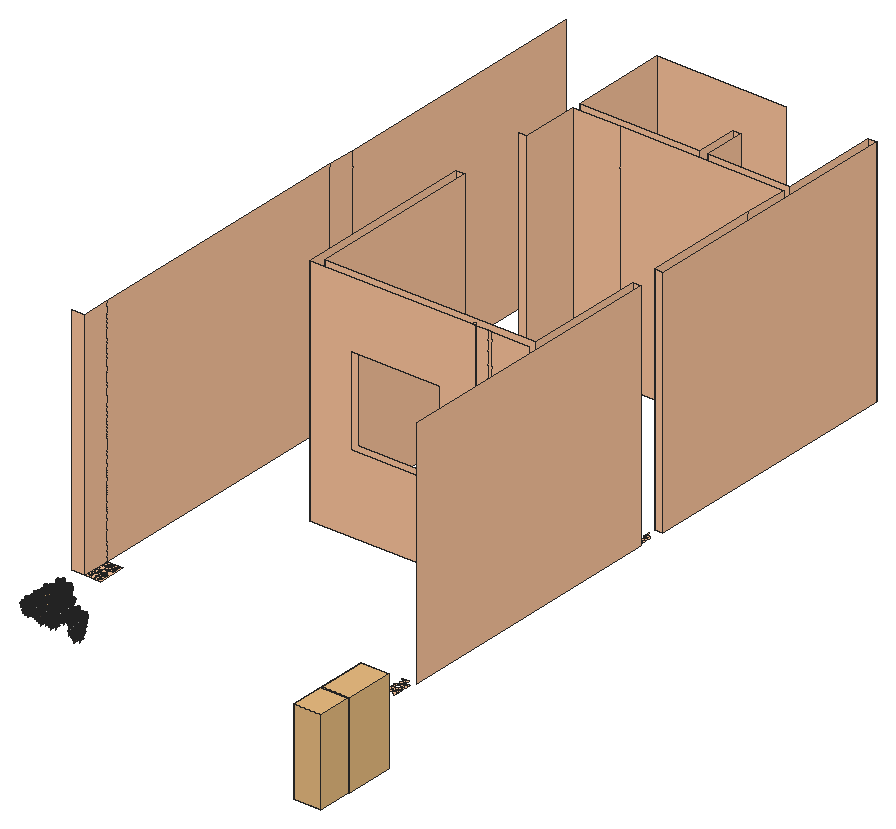
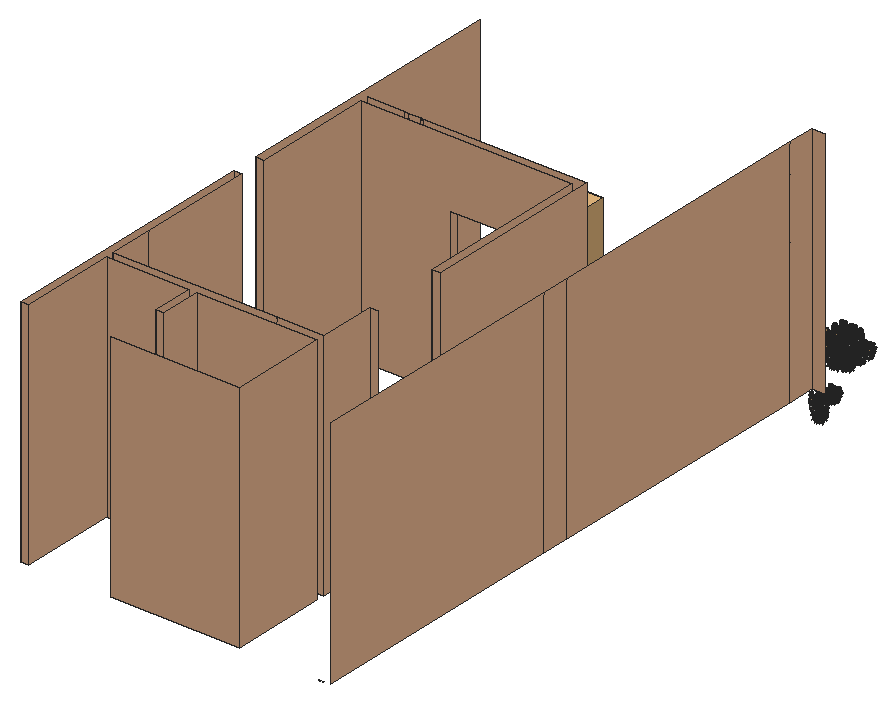
# SketchUp Ruby script. Lengths in inches.
U = 1.inch
M = Sketchup.active_model
def pt(a) = Geom::Point3d.new(a.map { |v| v * U })
def face(e, loops, mat)
  f = e.add_face(loops[0].map { |a| pt(a) })
  loops[1..].each { |l| e.add_face(l.map { |a| pt(a) }).erase! }
  f.material = f.back_material = mat if mat
  f
end
# faces: each face lists its corners as indices into pts; further lists are holes
def faces(e, pts, list, mat = nil) = list.each { |f| face(e, (f[0].is_a?(Array) ? f : [f]).map { |l| l.map { |i| pts[i] } }, mat) }
# xy, xz, yz: faces in a plane at the given z, y or x. An outline is a flat list of corners, or four numbers for a rectangle; further outlines are holes
def ring(l) = l.size == 4 ? [[l[0], l[1]], [l[2], l[1]], [l[2], l[3]], [l[0], l[3]]] : l.each_slice(2).to_a
def flat(e, list, mat, &to3) = list.each { |f| face(e, (f[0].is_a?(Array) ? f : [f]).map { |l| ring(l).map { |u, v| to3.(u, v) } }, mat) }
def xy(e, z, list, mat = nil) = flat(e, list, mat) { |x, y| [x, y, z] }
def xz(e, y, list, mat = nil) = flat(e, list, mat) { |x, z| [x, y, z] }
def yz(e, x, list, mat = nil) = flat(e, list, mat) { |y, z| [x, y, z] }
def lines(e, pts, list) = list.each { |a, b| e.add_line(pt(pts[a]), pt(pts[b])) }
# prism: a flat outline (further loops are holes) pulled along v
def prism(e, loops, v, mat = nil)
  f = face(e, loops, mat); d = Geom::Vector3d.new(v.map { |x| x * U })
  f.pushpull(f.normal.samedirection?(d) ? d.length : -d.length)
end
def box(e, o, s, mat = nil) = prism(e, [[o, [o[0] + s[0], o[1], o[2]], [o[0] + s[0], o[1] + s[1], o[2]], [o[0], o[1] + s[1], o[2]]]], [0, 0, s[2]], mat)
def at(x, y, z, deg = 0) = Geom::Transformation.translation(pt([x, y, z])) * Geom::Transformation.rotation(ORIGIN, Z_AXIS, deg.degrees)
def axes(o, x, y, z) = Geom::Transformation.new([*x, 0, *y, 0, *z, 0, *pt(o).to_a, 1])
def part(name) = M.definitions.add(name)
# library, detail: a bought-in or finely detailed component or shape, given as its bounding box
def library(name, o, s) = part(name).tap { |d| box(d.entities, o, s) }
def detail(e, o, s) = box(e.add_group.entities, o, s)
def put(e, d, t, mat = nil) = e.add_instance(d, t).tap { |i| i.material = mat if mat }
def group(e, t, mat = nil) = e.add_group.tap { |g| g.transformation = t; g.material = mat if mat }.entities
root = M.entities
M.materials.add("Vegetation_Bark_Crabapple").color = [91, 75, 65]
M.materials.add("[Color A02]1").color = [252, 197, 157]
M.materials.add("pollen").color = [217, 178, 104]
c1 = library("House+plant_10",[-33.59,-33.81,-21.29],[25.63,26.45,46.04])
c2 = part("Plane.002")
p = [[-2.92,82.99,124.67],[-2.92,-0.79,0],[2.92,-0.79,0],[2.92,82.99,124.67],[2.92,149.28,292.15],[-2.92,149.28,292.15],
  [2.92,182.43,464.87],[-2.92,182.43,464.87]]
faces(c2.entities,p,[[0,1,2,3],[3,4,5,0],[4,6,7,5]],"Vegetation_Bark_Crabapple")
c3 = part("Plane.003")
p = [[-13.75,10.1875,13.53],[-8.85,45.75,19.16],[-0.05,76.91,20.56],[0.09,-0.03,-0.02],[7.48,49.37,17.16],[14.16,9.16,9.9]]
faces(c3.entities,p,[[0,1,2,3],[4,5,3,2]])
c4 = part("Flower-123")
p = [[0.126,0.257,0.449],[0.155,0.204,0.548],[0.127,0.213,0.555],[0.093,0.267,0.458],[0.188,0.133,0.622],[0.183,0.129,0.631],
  [0.175,0.131,0.633],[0.165,0.14,0.628]]
faces(c4.entities,p,[[0,1,2,3],[1,4,5,6,7,2]],"pollen")
detail(c4.entities,[0,0,0],[0.33,0.41,0.7])
c5 = part("Group\#22")
put(c5.entities,c2,axes([0.24,0.01,0.18],[0.00584,-0.00173,-0.00142],[0.00119,0.00873,-0.00832],[0.00331,0.00566,0.01028]))
put(c5.entities,c3,axes([1.52,3.22,2.1875],[-0.00804,0.00596,-0.00897],[-0.00946,-0.00546,0.00721],[-0.0004,0.00943,0.00985]))
put(c5.entities,c3,axes([1.32,2.77,1.78],[0.01256,0.00031,-0.00351],[-0.00251,0.0076,-0.01232],[0.00145,0.0104,0.00911]))
put(c5.entities,c3,axes([1.78,3.75,2.82],[0.00359,0.00823,-0.01047],[-0.01158,0.00445,-0.0007],[0.0027,0.00817,0.01092]))
put(c5.entities,c3,axes([0.88,1.77,1.02],[0.01086,-0.00723,-0.00215],[0.00311,0.00724,-0.01286],[0.00676,0.00828,0.00937]))
put(c5.entities,c3,axes([1.72,3.66,2.68],[-0.00696,-0.00525,0.00789],[0.00768,-0.00731,0.00284],[0.00323,0.00607,0.01024]))
put(c5.entities,c3,axes([0.98,1.92,1.1],[-0.00641,-0.00676,0.01252],[0.01063,-0.00886,0.00097],[0.00617,0.00824,0.01132]))
put(c5.entities,c3,axes([1.42,3.04,1.99],[0.00101,-0.00541,0.01232],[0.01133,-0.00105,-0.00207],[0.00173,0.0101,0.00638]))
put(c5.entities,c3,axes([0.59,1,0.65],[0.0051,-0.00438,-0.01381],[-0.00968,0.00594,-0.00813],[0.00732,0.01091,-0.00112]))
put(c5.entities,c3,axes([1.1,2.28,1.42],[0.00541,0.00553,-0.01038],[-0.00976,0.00548,-0.00323],[0.00278,0.00847,0.00887]))
put(c5.entities,c3,axes([0.66,1.2,0.69],[0.00787,-0.0076,0.01038],[0.01088,0.00189,-0.01021],[0.00343,0.01143,0.00859]))
put(c5.entities,c3,axes([1,2.02,1.23],[-0.00332,0.0113,-0.00638],[-0.00988,0.0009,0.01004],[0.00758,0.00613,0.01028]))
put(c5.entities,c3,axes([1.58,3.35,2.32],[0.00647,0.00472,-0.01261],[-0.01005,0.00792,-0.00326],[0.0053,0.00927,0.0092]))
put(c5.entities,c3,axes([1.62,3.49,2.49],[0.0094,-0.00757,0.00183],[0.00666,0.00678,-0.00925],[0.00388,0.00669,0.01145]))
put(c5.entities,c3,axes([1.21,2.52,1.61],[-0.01302,0.00172,-0.00109],[-0.0017,-0.00726,0.01324],[0.00092,0.01085,0.00902]))
put(c5.entities,c3,axes([1.125,2.36,1.48],[0.00721,-0.01079,0.00269],[0.00807,0.00338,-0.01201],[0.0075,0.00674,0.01032]))
put(c5.entities,c3,axes([1.9,4,3.09],[0.00001,-0.00487,0.01359],[0.01166,-0.00316,-0.0017],[0.00346,0.01068,0.00569]))
put(c5.entities,c4,axes([2.27,4.3,3.3125],[-0.76505,0.00149,-0.64397],[-0.61285,-0.30881,0.72736],[-0.19778,0.95112,0.23716]))
put(c5.entities,c3,axes([0.67,1.42,0.8125],[0.00418,-0.00177,-0.01289],[-0.00136,0.01117,-0.00294],[0.01063,0.00213,0.0047]))
put(c5.entities,c3,axes([0.36,1.36,0.75],[0.00559,0.00872,-0.00936],[-0.00135,0.00895,0.0112],[0.01154,-0.00318,0.00584]))
put(c5.entities,c3,axes([1.13,1.46,0.92],[0.00037,0.00449,-0.01599],[-0.00588,0.01192,0.00478],[0.01254,0.00546,0.00271]))
put(c5.entities,c4,axes([1.91,4.52,3.45],[-0.75636,-0.57556,0.31088],[0.59252,-0.80417,-0.04724],[0.27718,0.14847,0.94928]))
put(c5.entities,c4,axes([2.12,4.17,3.27],[0.01541,0.99987,-0.00371],[-0.66505,0.01302,0.74668],[0.74664,-0.00904,0.66517]))
put(c5.entities,c4,axes([2.05,4.17,3.1875],[0.05514,0.99835,0.01633],[-0.20485,-0.0047,0.97878],[0.97724,-0.05731,0.20425]))
put(c5.entities,c4,axes([1.95,4.53,3.51],[-0.67965,-0.57263,0.45843],[0.47474,-0.81981,-0.32021],[0.55919,0,0.82904]))
put(c5.entities,c4,axes([2.12,4.37,3.18],[-0.03684,0.90233,0.42946],[-0.20892,-0.42721,0.87968],[0.97724,-0.05731,0.20425]))
put(c5.entities,c4,axes([1.99,3.97,3.47],[0.82904,0,-0.55919],[0,1,0],[0.55919,0,0.82904]))
put(c5.entities,c4,axes([2,3.97,3.43],[0.66131,0,0.75011],[0,1,0],[-0.75011,0,0.66131]))
put(c5.entities,c4,axes([2.28,4.28,3.48],[-0.2877,-0.35709,-0.88866],[-0.91973,-0.15572,0.36033],[-0.26705,0.921,-0.28363]))
put(c5.entities,c4,axes([1.95,4.53,3.46],[-0.85707,-0.51463,-0.02405],[0.51016,-0.85429,0.09964],[-0.07183,0.07313,0.99473]))
put(c5.entities,c4,axes([1.98,4.0625,3.66],[0.10005,0.76886,0.63153],[0.20466,0.60524,-0.76928],[-0.97371,0.20622,-0.0968]))
put(c5.entities,c4,axes([2.21,4.21,3.28],[0.01107,0.99991,-0.00785],[-0.71534,0.01341,0.69865],[0.69869,-0.00211,0.71542]))
put(c5.entities,c4,axes([1.86,4.48,3.42],[-0.09798,-0.20201,0.97447],[0.64597,-0.75778,-0.09214],[0.75705,0.62045,0.20474]))
put(c5.entities,c4,at(2.25,4.35,3.46,120))
put(c5.entities,c4,at(2.02,3.96,3.47))
put(c5.entities,c4,axes([2.1875,4.32,3.26],[-0.2678,0.91122,0.31298],[-0.60895,-0.41181,0.67793],[0.74664,-0.00904,0.66517]))
put(c5.entities,c4,axes([2.03,4.02,3.45],[0.99756,0,-0.06976],[0,1,0],[0.06976,0,0.99756]))
put(c5.entities,c4,axes([2.05,3.99,3.41],[0.19766,0,0.98027],[0,1,0],[-0.98027,0,0.19766]))
put(c5.entities,c4,axes([2.1,4.34,3.72],[-0.09883,0.86603,-0.49014],[-0.17118,-0.5,-0.84894],[-0.98027,0,0.19766]))
put(c5.entities,c4,axes([2.18,4.47,3.53],[0.15137,-0.29348,-0.9439],[-0.69645,-0.7093,0.10885],[-0.70146,0.64091,-0.31176]))
put(c5.entities,c4,axes([2.27,4.23,3.62],[-0.07449,0.99629,-0.04301],[-0.86282,-0.08601,-0.49815],[-0.5,0,0.86603]))
put(c5.entities,c4,axes([1.9,4.51,3.47],[-0.18374,-0.30318,0.93505],[0.54752,-0.82159,-0.1588],[0.81637,0.48278,0.31695]))
put(c5.entities,c4,axes([2.34,4.27,3.47],[-0.11925,0.65296,-0.74794],[-0.99139,-0.11938,0.05384],[-0.05413,0.74792,0.66158]))
put(c5.entities,c4,axes([2.03,4,3.41],[0.86603,0,0.5],[0,1,0],[-0.5,0,0.86603]))
put(c5.entities,c4,axes([1.77,4.36,3.36],[-0.17823,-0.16506,0.97005],[0.98053,-0.11233,0.16104],[0.08239,0.97987,0.18187]))
put(c5.entities,c4,axes([2.2,4.25,3.24],[-0.61909,0.78366,0.05103],[-0.23541,-0.24718,0.93994],[0.74921,0.56989,0.33751]))
put(c5.entities,c4,axes([2.1,4.2,3.19],[-0.58355,0.81023,0.05471],[0.17622,0.06058,0.98249],[0.79273,0.58297,-0.17813]))
put(c5.entities,c4,axes([1.78,4.42,3.35],[-0.12701,-0.00833,0.99187],[0.91049,-0.39772,0.11325],[0.39354,0.91747,0.05809]))
put(c5.entities,c4,axes([1.97,4.33,3.18],[-0.45394,0.75959,0.46579],[0.40685,-0.28839,0.86678],[0.79273,0.58297,-0.17813]))
put(c5.entities,c4,axes([2.2,4.22,3.68],[0.6255,-0.22092,-0.74829],[-0.6737,0.33082,-0.66082],[0.39354,0.91747,0.05809]))
put(c5.entities,c4,axes([2.2,4.05,3.41],[0.46326,0.30792,0.83101],[-0.67387,0.7314,0.10465],[-0.57558,-0.60847,0.54632]))
put(c5.entities,c4,axes([2.09,4.46,3.69],[-0.81522,0.47946,-0.32488],[-0.06426,-0.63237,-0.772],[-0.57558,-0.60847,0.54632]))
put(c5.entities,c4,axes([1.79,4.38,3.33],[-0.28578,-0.47426,0.83271],[0.95001,-0.02622,0.31111],[-0.12572,0.88,0.45804]))
put(c5.entities,c4,axes([2.17,4.34,3.73],[-0.71122,0.70221,0.03278],[-0.40358,-0.36968,-0.83693],[-0.57558,-0.60847,0.54632]))
put(c5.entities,c4,axes([2.2,4.2,3.3],[-0.66528,0.3275,-0.67093],[-0.55383,0.38617,0.73766],[0.50067,0.86233,-0.07553]))
put(c5.entities,c4,axes([1.76,4.3,3.4],[0.04081,0.76243,0.64579],[0.98982,-0.11906,0.07802],[0.13637,0.63603,-0.75952]))
put(c5.entities,c4,axes([2.13,4.49,3.52],[-0.95264,0.30339,0.02075],[-0.30229,-0.93732,-0.17336],[-0.03315,-0.17142,0.98464]))
put(c5.entities,c4,axes([2.25,4,3.45],[0.70641,0.60197,-0.37232],[-0.62885,0.77519,0.06021],[0.32487,0.1916,0.92615]))
put(c5.entities,c4,axes([2.11,4.21,3.23],[-0.81906,0.48983,-0.29868],[-0.18829,0.26227,0.94645],[0.54194,0.83143,-0.12259]))
put(c5.entities,c4,axes([2.2,4.23,3.61],[0.73847,0.26741,-0.61899],[-0.6737,0.33082,-0.66082],[0.02806,0.90501,0.42446]))
put(c5.entities,c4,axes([2.22,4.11,3.4],[0.1134,-0.03757,0.99284],[-0.67387,0.7314,0.10465],[-0.7301,-0.68091,0.05762]))
put(c5.entities,c4,axes([2.01,4.35,3.75],[-0.64029,0.6522,-0.40579],[0.23873,-0.33316,-0.91215],[-0.7301,-0.68091,0.05762]))
put(c5.entities,c4,axes([2.21,4.39,3.67],[-0.72493,0.6869,0.0515],[-0.56238,-0.54702,-0.62008],[-0.39776,-0.47848,0.78285]))
put(c5.entities,c4,axes([1.76,4.37,3.375],[0.04655,0.66582,0.74466],[0.96165,-0.23158,0.14695],[0.27029,0.70926,-0.65107]))
put(c5.entities,c4,axes([2.25,4.43,3.28],[-0.5104,-0.48462,-0.71038],[-0.65311,-0.31894,0.68683],[-0.55942,0.81451,-0.15373]))
put(c5.entities,c4,axes([2.28,4.65,3.33],[-0.5104,-0.48462,-0.71038],[-0.65311,-0.31894,0.68683],[-0.55942,0.81451,-0.15373]))
c6 = part("Group\#23")
put(c6.entities,c5,axes([5.13,2.49,1.91],[-0.108,0.99415,0],[-0.70297,-0.07637,0.70711],[0.70297,0.07637,0.70711]))
put(c6.entities,c5,axes([5.13,2.49,1.08],[-0.108,0.99415,0],[-0.70297,-0.07637,0.70711],[0.70297,0.07637,0.70711]))
put(c6.entities,c5,axes([4.47,2.97,0.4375],[-0.60599,-0.79547,0],[0.56248,-0.4285,0.70711],[-0.56248,0.4285,0.70711]))
put(c6.entities,c5,axes([4.94,2.86,-0.05],[0.00524,-0.99999,0],[0.7071,0.0037,0.70711],[-0.7071,-0.0037,0.70711]))
put(c6.entities,c5,axes([2.93,5.37,1.01],[-0.68962,0.72417,0],[-0.51207,-0.48763,0.70711],[0.51207,0.48763,0.70711]))
put(c6.entities,c5,axes([2.93,4.82,-0.05],[-0.98823,0.15299,0],[-0.10818,-0.69878,0.70711],[0.10818,0.69878,0.70711]))
put(c6.entities,c5,axes([6.18,5.29,1.13],[1,0,0],[0,0.70711,0.70711],[0,-0.70711,0.70711]))
put(c6.entities,c5,axes([3.49,6.03,1.01],[-0.108,0.99415,0],[-0.70297,-0.07637,0.70711],[0.70297,0.07637,0.70711]))
put(c6.entities,c5,axes([6.37,4.16,-0.13],[0.94495,-0.32722,0],[0.23138,0.66818,0.70711],[-0.23138,-0.66818,0.70711]))
put(c6.entities,c5,axes([5.84,5.86,0.11],[0.79441,0.60738,0],[-0.42948,0.56174,0.70711],[0.42948,-0.56174,0.70711]))
put(c6.entities,c5,axes([4.7,6.09,0.1875],[0.25882,0.96593,0],[-0.68301,0.18301,0.70711],[0.68301,-0.18301,0.70711]))
put(c6.entities,c5,axes([3.28,3.87,0.07],[-0.96456,-0.26387,0],[0.18659,-0.68205,0.70711],[-0.18659,0.68205,0.70711]))
put(c6.entities,c5,axes([5.96,3.21,1.01],[0.54902,-0.83581,0],[0.59101,0.38822,0.70711],[-0.59101,-0.38822,0.70711]))
put(c6.entities,c5,axes([4.45,5.31,1.53],[-0.0715,-0.99744,0],[0.7053,-0.05056,0.70711],[-0.7053,0.05056,0.70711]))
put(c6.entities,c5,axes([3.99,3.86,0.1875],[0.00524,-0.99999,0],[0.7071,0.0037,0.70711],[-0.7071,-0.0037,0.70711]))
put(c6.entities,c5,axes([3.84,4.21,0.1875],[-0.60599,-0.79547,0],[0.56248,-0.4285,0.70711],[-0.56248,0.4285,0.70711]))
put(c6.entities,c5,axes([4.45,5.67,0.1875],[-0.0715,-0.99744,0],[0.7053,-0.05056,0.70711],[-0.7053,0.05056,0.70711]))
put(c6.entities,c5,axes([4.68,4.3,0.1875],[0.54902,-0.83581,0],[0.59101,0.38822,0.70711],[-0.59101,-0.38822,0.70711]))
put(c6.entities,c5,axes([3.9,4.47,0.1875],[-0.96456,-0.26387,0],[0.18659,-0.68205,0.70711],[-0.18659,0.68205,0.70711]))
put(c6.entities,c5,axes([5.41,4.87,0.1875],[0.25882,0.96593,0],[-0.68301,0.18301,0.70711],[0.68301,-0.18301,0.70711]))
put(c6.entities,c5,axes([4.68,3.97,0.1875],[0.79441,0.60738,0],[-0.42948,0.56174,0.70711],[0.42948,-0.56174,0.70711]))
put(c6.entities,c5,axes([5.06,3.625,0.1875],[0.94495,-0.32722,0],[0.23138,0.66818,0.70711],[-0.23138,-0.66818,0.70711]))
put(c6.entities,c5,axes([4.64,4.71,0.1875],[-0.108,0.99415,0],[-0.70297,-0.07637,0.70711],[0.70297,0.07637,0.70711]))
put(c6.entities,c5,axes([5.34,4.26,0.1875],[1,0,0],[0,0.70711,0.70711],[0,-0.70711,0.70711]))
put(c6.entities,c5,axes([4.02,5.27,0.1875],[-0.98823,0.15299,0],[-0.10818,-0.69878,0.70711],[0.10818,0.69878,0.70711]))
put(c6.entities,c5,axes([4.38,5.37,0.1875],[-0.68962,0.72417,0],[-0.51207,-0.48763,0.70711],[0.51207,0.48763,0.70711]))
c7 = part("Kukka-altaaat")
put(c7.entities,c6,at(36.02,12.82,2.28))
put(c7.entities,c6,at(36.02,19.85,2.28))
put(c7.entities,c6,at(36.02,7.07,2.28))
put(c7.entities,c6,at(41.52,7.07,2.28))
put(c7.entities,c6,at(41.52,12.76,2.28))
put(c7.entities,c6,at(34.29,32.17,-7.59))
xy(root,-0.11,[[[7.86,46.0625,16.85,61.13],[15.83,48.22,15.65,48.4,15.83,48.6,15.83,49.99,15.65,50.17,15.83,50.37,15.83,51.76,15.65,51.95,14.77,51.05,15.65,50.17,13.91,48.37,13.02,49.26,12.13,50.14,11.25,51.02,10.375,51.9,11.25,52.8,12.13,51.92,13.01,52.8125,13.89,53.71,13.01,54.58,12.13,55.46,13.01,56.36,13.89,55.48,13.01,54.58,13.89,53.71,15.65,51.95,15.83,52.14],[11.25,52.8,10.375,53.67,9.5,54.55,10.39,55.43,11.28,56.32,12.13,55.46,11.25,54.57,10.39,55.43,9.5,54.55,8.87,53.91,8.87,60.12,9.25,60.12,9.5,59.86,8.87,59.23,8.87,58.73,9.5,58.09,8.87,57.46,8.87,56.95,9.5,56.32,8.87,55.6875,8.87,55.18,9.5,54.55,10.375,53.67,11.25,54.57,12.13,53.69],[8.87,47.08,8.87,48.09,9.5,47.46,9.12,47.08,9.88,47.08,9.5,47.46,10.375,48.35,11.27,47.46,10.9,47.08],[11.28,56.32,10.39,57.21,11.28,58.09,12.16,57.21],[13.01,56.36,12.16,57.21,13.05,58.09,13.89,57.25],[9.5,51.01,8.87,51.63,8.87,52.14,9.5,52.78,10.375,51.9],[14.77,58.15,13.93,58.98,14.82,59.86,15.65,59.04],[12.67,47.08,13.04,47.46,13.43,47.08],[14.82,59.86,14.57,60.12,15.07,60.12]],[8.87,47.08,9.12,47.08,9.5,47.46,8.87,48.09],[9.88,47.08,10.9,47.08,11.27,47.46,10.375,48.35,9.5,49.23,10.375,50.13,11.25,49.25,12.13,50.14,11.25,51.02,10.375,50.13,9.5,51.01,8.87,51.63,8.87,50.37,9.5,51.01,8.87,50.37,8.87,49.86,9.5,49.23,10.375,50.13,11.25,49.25,12.15,48.36,13.04,47.46,13.91,48.37,14.8,47.47,14.44,47.08,13.43,47.08,13.04,47.46,12.67,47.08,15.83,47.08,15.83,48.22,14.78,49.27,13.91,48.37,13.02,49.26,12.15,48.36,11.25,49.25,10.375,48.35,9.5,47.46],[9.88,47.08,10.9,47.08,11.27,47.46,10.375,48.35,9.5,47.46],[12.67,47.08,13.43,47.08,13.04,47.46],
  [14.44,47.08,15.2,47.08,14.8,47.47],[15.2,47.08,15.83,47.08,15.83,48.22,15.65,48.4,14.8,47.47],[174.25,47.08,174.88,47.08,174.88,48.22,174.7,48.4,173.82,49.27,172.95,48.37,172.07,49.26,171.18,50.14,170.3,49.25,171.19,48.36,172.07,49.26,172.94,50.15,173.82,49.27,174.7,48.4,173.85,47.47],[13.04,47.46,13.91,48.37,13.02,49.26,12.15,48.36],[14.8,47.47,15.65,48.4,13.9,50.15,14.77,51.05,13.89,51.93,13.01,52.8125,12.13,51.92,13.9,50.15,13.02,49.26,13.91,48.37],
  [15.83,48.22,15.83,48.6,15.65,48.4],[15.83,48.22,15.83,48.6,15.65,48.4],[10.375,48.35,11.25,49.25,10.375,50.13,9.5,49.23],[169.42,48.35,170.3,49.25,169.42,50.13,168.54,49.23],[171.19,48.36,172.07,49.26,171.18,50.14,170.3,49.25],
  [172.95,48.37,173.82,49.27,172.94,50.15,172.07,49.26],[8.87,48.6,8.87,49.86,9.5,49.23,10.375,50.13,9.5,51.01,8.87,50.37,8.87,49.86,9.5,49.23],[8.87,48.6,9.5,49.23,8.87,49.86],[11.25,49.25,12.13,50.14,11.25,51.02,10.375,50.13],[13.02,49.26,13.9,50.15,13.01,51.04,13.89,51.93,14.77,52.83,15.65,53.72,15.83,53.91,15.83,60.12,15.07,60.12,14.82,59.86,15.65,59.04,15.83,59.23,15.83,58.85,15.65,59.04,14.77,58.15,13.89,57.25,13.05,58.09,13.93,58.98,14.82,59.86,14.57,60.12,11.53,60.12,11.28,59.86,10.39,58.98,9.5,58.09,10.39,57.21,9.5,56.32,8.87,56.95,8.87,55.6875,9.5,56.32,10.39,57.21,11.28,58.09,10.39,58.98,9.5,59.86,9.76,60.12,9.25,60.12,9.5,59.86,10.39,58.98,11.28,58.09,12.16,58.98,11.28,59.86,13.05,58.09,12.16,57.21,13.01,56.36,13.89,57.25,15.65,55.49,14.77,54.6,13.89,55.48,14.77,56.37,15.65,55.49,15.83,55.6875,15.83,55.31,15.65,55.49,14.77,54.6,15.65,53.72,14.77,52.83,15.65,51.95,14.77,51.05,13.89,51.93,13.01,51.04,12.13,50.14],
  [13.02,49.26,13.9,50.15,13.01,51.04,12.13,50.14],[14.78,49.27,15.65,50.17,14.77,51.05,13.9,50.15],[173.82,49.27,174.69,50.17,173.82,51.05,172.94,50.15],[15.83,49.99,15.83,50.37,15.65,50.17],[174.88,49.99,174.69,50.17,174.88,50.37,174.88,51.76,174.69,51.95,173.82,51.05,172.93,51.93,172.06,51.04,172.94,50.15,173.82,51.05,174.69,51.95,174.88,52.14],
  [169.42,50.13,170.3,51.02,169.42,51.9,168.54,51.01,167.91,50.37,167.91,51.63,168.54,51.01],[12.13,50.14,13.01,51.04,12.13,51.92,11.25,51.02],[171.18,50.14,172.06,51.04,171.18,51.92,170.3,51.02],[8.87,50.37,9.5,51.01,8.87,51.63],[9.5,51.01,10.375,51.9,9.5,52.78,8.87,52.14,8.87,51.63],
  [11.25,51.02,12.13,51.92,11.25,52.8,10.375,51.9],[170.3,51.02,171.18,51.92,170.3,52.8,169.42,51.9],[172.06,51.04,172.93,51.93,172.06,52.8125,171.18,51.92],[14.77,51.05,15.65,51.95,14.77,52.83,13.89,51.93],[15.83,51.76,15.83,52.14,15.65,51.95],
  [169.42,51.9,170.3,52.8,169.42,53.67,168.54,52.78],[13.89,51.93,14.77,52.83,13.89,53.71,13.01,52.8125],[172.93,51.93,173.8125,52.83,172.93,53.71,172.06,52.8125],[8.87,52.14,9.5,52.78,10.375,53.67,11.25,52.8,13.01,54.58,13.89,53.71,14.77,54.6,13.89,55.48,14.77,54.6,15.65,55.49,14.77,56.37,15.65,57.27,14.77,58.15,15.65,57.27,15.83,57.46,15.83,57.08,15.65,57.27,14.77,56.37,13.89,55.48,13.01,54.58,12.13,53.69,11.25,54.57,10.375,53.67,9.5,52.78,8.87,53.41],[8.87,52.14,9.5,52.78,8.87,53.41],
  [11.25,52.8,12.13,53.69,11.25,54.57,10.375,53.67],[173.8125,52.83,174.69,53.72,173.8125,54.6,172.93,53.71],[169.42,53.67,170.3,54.57,169.42,55.45,168.54,54.55],[169.42,53.67,170.3,54.57,171.18,55.46,170.3,56.34,171.17,57.24,170.32,58.09,169.43,57.21,170.3,56.34,169.42,55.45,168.54,54.55],[13.89,53.71,14.77,54.6,13.89,55.48,13.01,54.58],
  [172.93,53.71,173.8125,54.6,172.93,55.48,172.06,54.58],[15.65,53.72,15.83,53.91,15.83,55.31,15.65,55.49,14.77,54.6],[8.87,53.91,9.5,54.55,8.87,55.18],[11.25,54.57,12.13,55.46,11.28,56.32,10.39,55.43],[13.01,54.58,13.89,55.48,13.01,56.36,12.13,55.46],
  [172.06,54.58,172.93,55.48,172.06,56.36,171.18,55.46],[173.8125,54.6,174.69,55.49,173.8125,56.37,172.93,55.48],[15.65,55.49,15.83,55.6875,15.83,57.08,15.65,57.27,14.77,56.37],[8.87,55.6875,9.5,56.32,8.87,56.95],[11.28,56.32,12.16,57.21,11.28,58.09,10.39,57.21],
  [170.3,56.34,171.17,57.24,170.32,58.09,169.43,57.21],[13.01,56.36,13.89,57.25,13.05,58.09,12.16,57.21],[172.06,56.36,171.17,57.24,172.05,58.14,171.21,58.98,172.09,59.86,171.84,60.12,170.57,60.12,170.32,59.86,170.07,60.12,168.8,60.12,168.55,59.86,169.43,58.98,170.32,59.86,171.21,58.98,172.05,58.14,172.93,57.25],[172.06,56.36,172.93,57.25,172.05,58.14,171.17,57.24],[14.77,56.37,15.65,57.27,14.77,58.15,13.89,57.25],
  [173.8125,56.37,174.69,57.27,173.8125,58.15,172.93,57.25],[10.39,57.21,11.28,58.09,10.39,58.98,9.5,58.09],[15.65,57.27,15.83,57.46,15.83,58.85,15.65,59.04,14.77,58.15],[8.87,57.46,9.5,58.09,8.87,58.73],[11.28,58.09,12.16,58.98,11.28,59.86,10.39,58.98],
  [13.05,58.09,13.93,58.98,13.05,59.86,13.3,60.12,12.79,60.12,13.05,59.86,12.16,58.98],[170.32,58.09,171.21,58.98,170.32,59.86,169.43,58.98],[14.77,58.15,15.65,59.04,14.82,59.86,13.93,58.98],[12.16,58.98,13.05,59.86,12.79,60.12,11.53,60.12,11.28,59.86],[13.93,58.98,14.82,59.86,14.57,60.12,13.3,60.12,13.05,59.86],
  [15.65,59.04,15.83,59.23,15.83,60.12,15.07,60.12,14.82,59.86],[8.87,59.23,9.5,59.86,9.25,60.12,8.87,60.12],[9.5,59.86,9.76,60.12,9.25,60.12],[14.82,59.86,15.07,60.12,14.57,60.12],[[7.86,212.2,16.85,227.14],[8.87,213.21,8.87,223.09,9.51,222.44,10.39,221.54,11.25,220.66,12.13,219.77,13.01,218.87,12.13,217.99,11.25,218.89,12.13,219.77,11.25,220.66,10.375,219.78,9.5,220.67,10.39,221.54,9.51,222.44,8.87,221.82,8.87,221.32,9.5,220.67,8.87,220.05,8.87,219.54,9.5,218.91,8.87,218.28,8.87,217.77,9.5,217.14,8.87,216.5,8.87,216,9.5,215.36,8.87,214.73,8.87,214.22,9.5,213.59,9.12,213.21],[12.16,216.25,11.28,217.14,10.39,218.02,9.5,218.91,10.375,219.78,11.25,218.89,10.39,218.02,11.28,217.14,12.13,217.99,13.01,217.1],[13.87,221.51,12.98,222.39,13.87,223.28,14.76,222.39,15.64,223.28,14.76,224.16,15.64,225.05,15.83,225.24,15.83,223.09,15.64,223.28,14.76,222.39],[12.67,213.21,13.05,213.59,11.28,215.36,12.16,216.25,13.05,215.36,12.16,214.48,13.43,213.21],[10.39,214.48,9.5,215.36,10.39,216.25,11.28,215.36],[13.87,219.73,12.98,220.62,13.87,221.51,14.76,220.62],[13.89,217.98,13.01,218.87,13.87,219.73,14.76,218.85],[9.88,213.21,9.5,213.59,10.39,214.48,11.28,213.59,10.9,213.21],[8.87,225.37,8.87,226.13,9.25,226.13,9.48,225.89],[14.44,213.21,15.83,214.6,15.83,214.22,15.65,214.42,14.82,213.59,15.2,213.21]],
  [8.87,213.21,9.12,213.21,9.5,213.59,8.87,214.22],[10.9,213.21,11.65,213.21,11.28,213.59,12.16,214.48,13.05,213.59,13.93,214.48,13.05,215.36,13.93,214.48,14.77,215.3125,13.89,216.21,14.77,215.3125,15.65,216.1875,14.77,217.08,15.65,216.1875,15.83,216.38,15.83,218.15,15.64,217.96,14.76,218.85,13.87,219.73,13.01,218.87,13.89,217.98,13.01,217.1,12.13,217.99,9.5,215.36,10.39,214.48,11.28,215.36,10.39,216.25,11.28,217.14,12.16,216.25,13.01,217.1,13.89,216.21,14.77,217.08,13.89,217.98,15.83,219.92,15.83,221.32,13.87,223.28,12.98,222.39,12.13,223.25,13.03,224.12,12.14,225,13.04,225.88,13.92,225,13.03,224.12,13.87,223.28,14.76,224.16,15.64,225.05,15.83,224.86,15.83,223.47,15.64,223.28,13.92,225,13.03,224.12,12.14,225,13.04,225.88,13.3,226.13,11.02,226.13,11.27,225.88,12.14,225,11.25,224.13,10.35,223.26,9.51,222.44,10.39,221.54,11.24,222.37,12.13,223.25,11.24,222.37,12.1,221.51,12.98,222.39,13.87,221.51,14.76,222.39,15.64,221.51,14.76,220.62,15.64,219.73,14.76,218.85,15.64,217.96,14.77,217.08,13.89,216.21,13.05,215.36,12.16,214.48,11.28,213.59],[9.88,213.21,10.9,213.21,11.28,213.59,10.39,214.48,9.5,213.59],[10.9,213.21,11.65,213.21,11.28,213.59],[12.67,213.21,13.43,213.21,13.05,213.59],
  [14.44,213.21,15.2,213.21,14.82,213.59],[13.05,213.59,13.93,214.48,13.05,215.36,12.16,214.48],[173.87,213.59,174.69,214.42,173.8125,215.3125,172.98,214.48],[15.83,214.22,15.83,214.6,15.65,214.42],[10.39,214.48,11.28,215.36,10.39,216.25,9.5,215.36],
  [12.16,214.48,13.05,215.36,12.16,216.25,11.28,215.36],[13.93,214.48,14.77,215.3125,13.89,216.21,13.05,215.36],[172.98,214.48,173.8125,215.3125,172.93,216.21,172.09,215.36],[8.87,214.73,9.5,215.36,8.87,216],[14.77,215.3125,15.65,216.1875,14.77,217.08,13.89,216.21],
  [173.8125,215.3125,174.69,216.1875,173.8125,217.08,172.93,216.21],[172.09,215.36,172.93,216.21,172.06,217.1,171.33,216.38,171.33,216.125],[15.83,216,15.65,216.1875,15.83,216.38,15.83,217.77,15.64,217.96,14.77,217.08,15.65,216.1875,15.83,216.38],[15.83,216,15.83,216.38,15.65,216.1875],[13.89,216.21,14.77,217.08,13.89,217.98,13.01,217.1],
  [172.93,216.21,173.8125,217.08,172.93,217.98,172.06,217.1],[12.16,216.25,13.01,217.1,12.13,217.99,11.28,217.14],[8.87,216.5,9.5,217.14,8.87,217.77],[173.8125,217.08,174.6875,217.96,173.8,218.85,172.93,217.98],[15.83,217.77,15.83,218.15,15.64,217.96],
  [15.64,217.96,15.83,218.15,15.83,219.54,15.64,219.73,14.76,218.85],[13.89,217.98,14.76,218.85,13.87,219.73,13.01,218.87],[172.93,217.98,173.8,218.85,172.92,219.73,172.06,218.87],[12.13,217.99,13.01,218.87,12.13,219.77,11.25,218.89],[10.39,218.02,11.25,218.89,10.375,219.78,9.5,218.91],
  [8.87,218.28,9.5,218.91,8.87,219.54],[173.8,218.85,174.6875,219.73,173.8,220.62,172.92,219.73],[15.83,219.54,15.83,219.92,15.64,219.73],[13.87,219.73,14.76,220.62,13.87,221.51,12.98,220.62],[15.64,219.73,15.83,219.92,15.83,221.32,15.64,221.51,14.76,220.62],
  [172.92,219.73,173.8,220.62,172.92,221.51,172.03,220.62],[12.13,219.77,12.98,220.62,12.1,221.51,11.25,220.66],[10.375,219.78,11.25,220.66,10.39,221.54,9.5,220.67],[171.33,219.92,172.03,220.62,171.33,221.32],[8.87,220.05,9.5,220.67,8.87,221.32],
  [13.87,221.51,14.76,222.39,13.87,223.28,12.98,222.39],[10.39,221.54,11.24,222.37,10.35,223.26,9.51,222.44],[171.33,221.7,172.03,222.39,171.33,223.09],[8.87,221.82,9.51,222.44,8.87,223.09],[11.24,222.37,12.13,223.25,11.25,224.13,10.35,223.26,9.45,224.15,8.87,223.6,8.87,224.73,9.45,224.15,10.35,223.26],
  [15.83,223.09,15.83,223.47,15.64,223.28],[12.13,223.25,13.03,224.12,12.14,225,11.25,224.13],[13.87,223.28,14.76,224.16,13.92,225,13.03,224.12],[15.64,223.28,15.83,223.47,15.83,224.86,15.64,225.05,14.76,224.16],[8.87,223.6,9.45,224.15,8.87,224.73],
  [13.03,224.12,13.92,225,13.04,225.88,12.14,225],[15.83,224.86,15.83,225.24,15.64,225.05],[12.14,225,13.04,225.88,12.79,226.13,11.53,226.13,11.27,225.88],[13.92,225,14.82,225.875,14.57,226.13,13.3,226.13,13.04,225.88],[10.36,225.02,11.27,225.88,11.02,226.13,9.76,226.13,9.48,225.89],
  [8.87,225.37,9.48,225.89,9.25,226.13,8.87,226.13],[14.82,225.875,15.07,226.13,14.57,226.13],[11.27,225.88,11.53,226.13,11.02,226.13],[13.04,225.88,13.3,226.13,12.79,226.13],[9.48,225.89,9.76,226.13,9.25,226.13],
  [10.9,372.26,11.65,372.26,11.28,372.64],[12.67,372.26,13.43,372.26,13.05,372.64]],"[Color A02]1")
xz(root,46.0625,[[0.89,-0.11,7.86,125.89]],"[Color A02]1")
xz(root,142.17,[[[52.81,-0.11,142.01,125.89],[75.18,41.89,123.18,89.89]],[142.01,-0.11,142.65,125.89],[142.65,-0.11,148.92,125.89],[148.92,-0.11,151.33,125.89],[151.33,-0.11,171.33,125.89]],"[Color A02]1")
xz(root,146.61,[[[57.37,-0.11,171.33,125.89],[75.18,41.89,123.18,89.89]]],"[Color A02]1")
xz(root,212.2,[[171.33,-0.11,175.89,125.89]],"[Color A02]1")
xz(root,227.14,[[171.33,-0.11,175.89,125.89]],"[Color A02]1")
xz(root,241.2,[[52.81,-0.11,57.37,125.89]],"[Color A02]1")
xz(root,283.24,[[52.81,-0.11,57.37,125.89]],"[Color A02]1")
xz(root,314.26,[[57.37,-0.11,82.82,125.89],[82.82,-0.11,171.33,125.89]],"[Color A02]1")
xz(root,318.69,[[57.37,-0.11,122.33,125.89],[126.89,-0.11,171.33,125.89]],"[Color A02]1")
xz(root,341.23,[[122.33,-0.11,126.89,125.89]],"[Color A02]1")
xz(root,371.24,[[57.37,-0.11,126.89,125.89],[171.33,-0.11,175.89,125.89]],"[Color A02]1")
yz(root,7.86,[[46.0625,-0.11,61.13,125.89],[61.13,-0.11,212.2,125.89],[212.2,-0.11,227.14,125.89],[227.14,-0.11,371.24,125.89]],"[Color A02]1")
yz(root,52.81,[[142.17,-0.11,241.2,125.89]],"[Color A02]1")
yz(root,57.37,[[146.61,-0.11,241.2,125.89],[283.24,-0.11,314.26,125.89],[318.69,-0.11,371.24,125.89]],"[Color A02]1")
yz(root,122.33,[[318.69,-0.11,341.23,125.89]],"[Color A02]1")
yz(root,126.89,[[318.69,-0.11,341.23,125.89]],"[Color A02]1")
yz(root,171.33,[[146.61,-0.11,212.2,125.89],[227.14,-0.11,290.2,125.89],[290.2,-0.11,314.26,125.89],[318.69,-0.11,371.24,125.89]],"[Color A02]1")
yz(root,175.89,[[61,-0.11,212.2,125.89],[227.14,-0.11,371.24,125.89]],"[Color A02]1")
p = [[142.01,142.17,-0.11],[140.6875,143.4375,-0.11],[140.6875,143.4375,125.89],[142.01,142.17,125.89],[141.07,143.82,-0.11],[142.65,142.17,-0.11],
  [142.65,142.17,125.89],[141.07,143.82,125.89]]
faces(root,p,[[0,1,2,3],[4,5,6,7],[1,4,7,2]],"[Color A02]1")
put(root,c1,axes([182.28,27.58,-9.78],[0.5829,0,0],[0,1,0],[0,0,1]))
put(root,c7,axes([-25.15,-3.14,-9.25],[1,0,0],[0,1,0],[0,0,2]))
put(root,c7,at(-31.77,-3.14,-4.99))
put(root,c1,axes([183.21,45.73,-9.16],[0.5829,0,0],[0,1,0],[0,0,1]))
